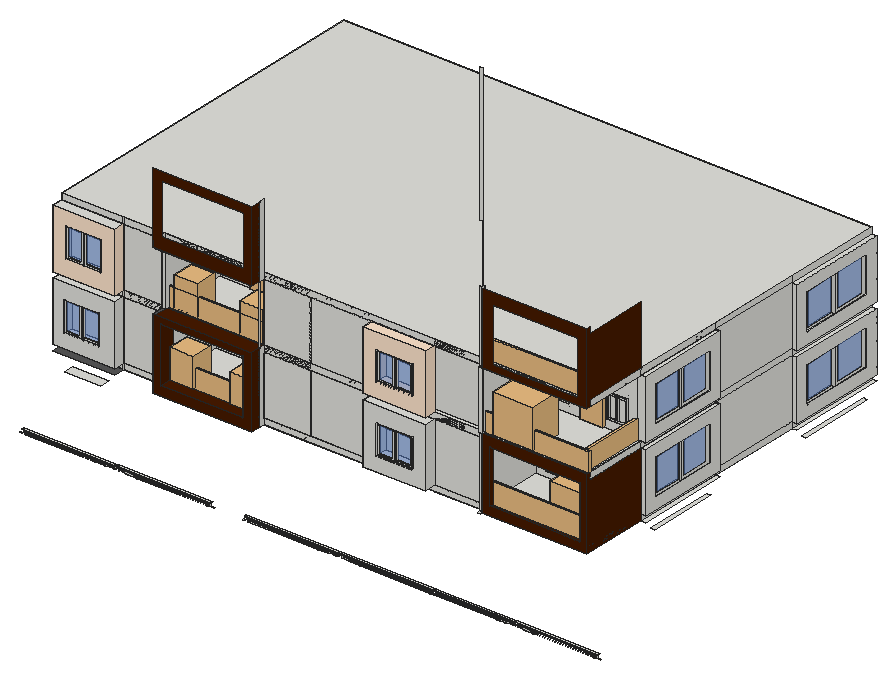
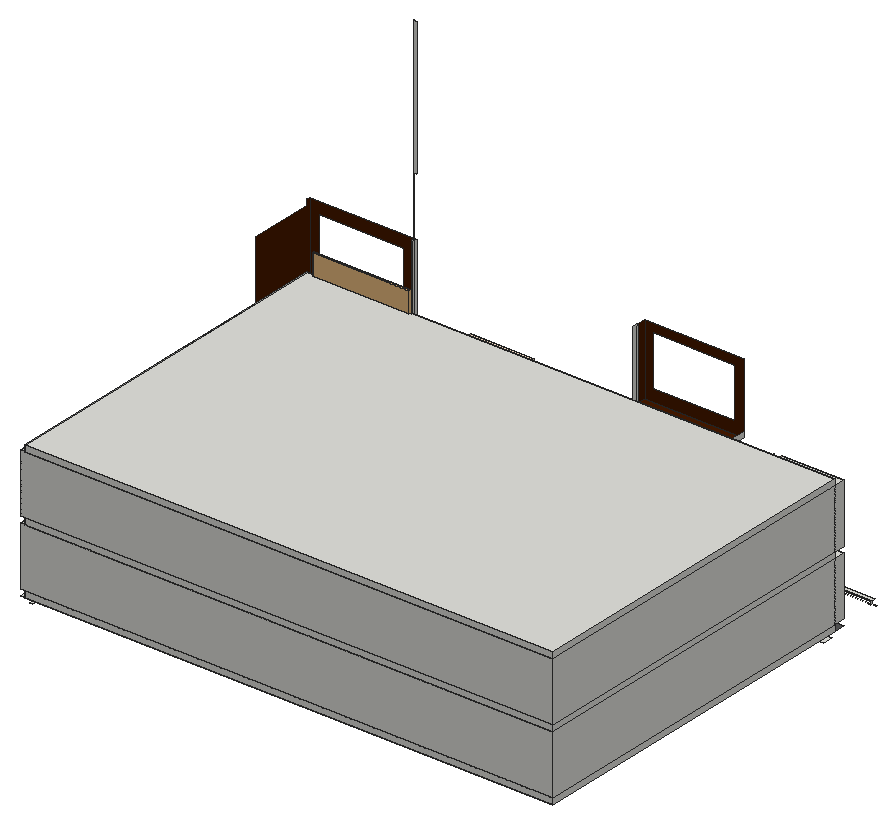
# SketchUp Ruby script. Lengths in inches.
U = 1.inch
M = Sketchup.active_model
def pt(a) = Geom::Point3d.new(a.map { |v| v * U })
def face(e, loops, mat)
  f = e.add_face(loops[0].map { |a| pt(a) })
  loops[1..].each { |l| e.add_face(l.map { |a| pt(a) }).erase! }
  f.material = f.back_material = mat if mat
  f
end
# faces: each face lists its corners as indices into pts; further lists are holes
def faces(e, pts, list, mat = nil) = list.each { |f| face(e, (f[0].is_a?(Array) ? f : [f]).map { |l| l.map { |i| pts[i] } }, mat) }
# xy, xz, yz: faces in a plane at the given z, y or x. An outline is a flat list of corners, or four numbers for a rectangle; further outlines are holes
def ring(l) = l.size == 4 ? [[l[0], l[1]], [l[2], l[1]], [l[2], l[3]], [l[0], l[3]]] : l.each_slice(2).to_a
def flat(e, list, mat, &to3) = list.each { |f| face(e, (f[0].is_a?(Array) ? f : [f]).map { |l| ring(l).map { |u, v| to3.(u, v) } }, mat) }
def xy(e, z, list, mat = nil) = flat(e, list, mat) { |x, y| [x, y, z] }
def xz(e, y, list, mat = nil) = flat(e, list, mat) { |x, z| [x, y, z] }
def yz(e, x, list, mat = nil) = flat(e, list, mat) { |y, z| [x, y, z] }
def lines(e, pts, list) = list.each { |a, b| e.add_line(pt(pts[a]), pt(pts[b])) }
# prism: a flat outline (further loops are holes) pulled along v
def prism(e, loops, v, mat = nil)
  f = face(e, loops, mat); d = Geom::Vector3d.new(v.map { |x| x * U })
  f.pushpull(f.normal.samedirection?(d) ? d.length : -d.length)
end
def box(e, o, s, mat = nil) = prism(e, [[o, [o[0] + s[0], o[1], o[2]], [o[0] + s[0], o[1] + s[1], o[2]], [o[0], o[1] + s[1], o[2]]]], [0, 0, s[2]], mat)
def at(x, y, z, deg = 0) = Geom::Transformation.translation(pt([x, y, z])) * Geom::Transformation.rotation(ORIGIN, Z_AXIS, deg.degrees)
def axes(o, x, y, z) = Geom::Transformation.new([*x, 0, *y, 0, *z, 0, *pt(o).to_a, 1])
def part(name) = M.definitions.add(name)
# library, detail: a bought-in or finely detailed component or shape, given as its bounding box
def library(name, o, s) = part(name).tap { |d| box(d.entities, o, s) }
def detail(e, o, s) = box(e.add_group.entities, o, s)
def put(e, d, t, mat = nil) = e.add_instance(d, t).tap { |i| i.material = mat if mat }
def group(e, t, mat = nil) = e.add_group.tap { |g| g.transformation = t; g.material = mat if mat }.entities
root = M.entities
M.materials.add("[Color C01]").color = [255, 229, 204]
M.materials.add("[Color C07]").color = [71, 27, 0]
M.materials.add("[Color M06]").color = [86, 86, 86]
M.materials.add("[Color_000]").color = [255, 255, 255]
M.materials.add("[Translucent Glass Blue]").color = [100, 149, 237]
M.materials["[Translucent Glass Blue]"].alpha = 0.5
c1 = library("porta 4",[0.2,-5.42,1.33],[46.55,4.72,83.21])
c2 = library("Glass balustrade section",[0,0,0],[60.75,3.875,44.35])
c3 = library("KentiaPalm",[-22.86,-14.31,0],[47.49,43.96,59.125])
c4 = library("Round Planter with Plant",[-35.48,-39.77,0],[80.62,63.55,77.875])
c5 = part("Window")
xy(c5.entities,31.72,[[-0.78,88.6,2.72,128.1]])
xy(c5.entities,34.95,[[-0.78,91.53,0.84,106.59],[0.84,91.53,1.05,97.58],[1.05,91.53,1.42,106.59],[1.42,91.53,2.72,106.59],[0.84,97.58,1.05,98.18],
  [0.84,98.18,1.05,106.59]])
xy(c5.entities,35.27,[[-0.78,110.09,0.97,125.14],[1.05,110.09,2.72,125.14]])
xy(c5.entities,58.35,[[2.72,108.74,3.8,109.74]])
xy(c5.entities,77.8125,[[-0.78,110.09,2.72,125.14],[0.97,110.09,1.05,125.14]])
xy(c5.entities,77.93,[[-0.78,91.53,0.84,106.59],[1.05,91.53,1.42,106.59],[1.42,91.53,2.72,106.59]])
xy(c5.entities,80.72,[[-0.78,88.6,2.72,128.1]])
xz(c5.entities,88.6,[[-0.78,31.72,2.72,80.72]])
xz(c5.entities,91.53,[[-0.78,34.95,0.84,77.93],[1.05,34.95,1.42,77.93],[1.42,34.95,2.72,77.93]])
xz(c5.entities,106.59,[[-0.78,34.95,0.84,77.93],[0.84,34.95,1.05,77.93],[0.84,34.95,2.72,77.93]])
xz(c5.entities,108.74,[[3.8,54.35,4.22,54.6,4.22,59.47,2.72,59.97,2.72,58.35,3.8,58.35]])
xz(c5.entities,109.74,[[3.8,54.35,3.8,58.35,2.72,58.35,2.72,59.97,4.22,59.47,4.22,54.6]])
xz(c5.entities,110.09,[[-0.78,35.27,0.97,77.8125],[1.05,35.27,2.72,77.8125]])
xz(c5.entities,125.14,[[-0.78,35.27,0.97,77.8125],[0.97,35.27,1.05,80.72],[1.05,35.27,2.72,77.8125]])
xz(c5.entities,128.1,[[-0.78,31.72,2.72,80.72]])
yz(c5.entities,-0.78,[[[88.6,31.72,128.1,80.72],[91.53,34.95,106.59,77.93],[110.09,35.27,125.14,77.8125]]])
yz(c5.entities,0.84,[[91.53,34.95,106.59,77.93]])
yz(c5.entities,0.97,[[110.09,35.27,125.14,77.8125]])
yz(c5.entities,1.05,[[91.53,34.95,106.59,77.93],[110.09,35.27,125.14,77.8125]])
yz(c5.entities,1.42,[[91.53,34.95,106.59,77.93]])
yz(c5.entities,2.72,[[[88.6,31.72,108.35,80.72],[91.53,34.95,106.59,77.93]],[[108.35,31.72,128.1,80.72],[110.09,35.27,125.14,77.8125],[108.74,58.35,109.74,59.97]]])
yz(c5.entities,3.8,[[108.74,54.35,109.74,58.35]])
yz(c5.entities,4.22,[[108.74,54.6,109.74,59.47]])
p = [[4.22,108.74,54.6],[3.8,108.74,54.35],[3.8,109.74,54.35],[4.22,109.74,54.6],[2.72,109.74,59.97],[2.72,108.74,59.97],
  [4.22,108.74,59.47],[4.22,109.74,59.47],[-0.78,86.4,89.94],[-0.78,86.44,89.94],[15.22,130.69,89.94],[15.22,130.65,89.94],
  [-0.78,86.44,28.19],[-0.78,86.4,28.19],[7.72,130.69,89.94],[7.72,130.65,89.94]]
faces(c5.entities,p,[[0,1,2,3],[4,5,6,7]])
lines(c5.entities,p,[[8,9],[10,11],[12,13],[14,15]])
c6 = part("Janela aluminio")
xy(c6.entities,0,[[0,0,47.24,1.57],[23.62,1.57,47.24,2.76],[0,2.76,25.98,3.9375],[0,3.9375,47.24,5.91]])
xy(c6.entities,43.31,[[0,0,47.24,1.57],[23.62,1.57,47.24,2.76],[0,2.76,0,5.91,47.24,5.91,47.24,3.9375,25.98,3.9375,25.98,2.76],[25.98,2.76,47.24,3.9375]])
xz(c6.entities,1.57,[[0,0,23.62,0,23.62,41.34,21.26,41.34,21.26,1.97,1.97,1.97,1.97,41.34,23.62,41.34,23.62,43.31,0,43.31],[[23.62,0,47.24,43.31],[25.7,1.97,45.28,41.34]]])
xz(c6.entities,2.76,[[[0,0,23.62,43.31],[2.36,2.36,21.26,40.94]],[23.62,0,25.98,43.31]])
xz(c6.entities,2.76,[[2.36,2.36,21.26,40.94]],"[Translucent Glass Blue]")
xz(c6.entities,3.9375,[[25.98,0,25.98,2.36,44.88,2.36,44.88,40.94,25.98,40.94,25.98,43.31,47.24,43.31,47.24,0]])
xz(c6.entities,3.9375,[[25.98,2.36,44.88,40.94]],"[Translucent Glass Blue]")
yz(c6.entities,0,[[0,0,1.57,43.31],[2.76,0,5.91,43.31]])
yz(c6.entities,23.62,[[1.57,0,2.76,43.31]])
yz(c6.entities,25.98,[[2.76,0,3.9375,43.31]])
yz(c6.entities,47.24,[[0,0,1.57,43.31],[1.57,0,2.76,43.31],[3.9375,0,5.91,43.31]])
xy(root,64.41,[[193.54,12.93,336.13,13.56],[336.13,12.93,354.73,13.56],[401.38,12.93,419.98,13.56],[419.98,12.93,562.58,13.56],[643.44,12.93,786.03,13.56],
  [786.03,12.93,804.64,13.56],[851.28,12.93,869.89,13.56],[869.89,12.93,1012.48,13.56],[1024.39,12.93,1148.45,13.56],[1148.45,12.93,1164.63,13.56],
  [1205.21,12.93,1221.4,13.56],[1221.4,12.93,1345.46,13.56],[193.54,13.81,336.13,14.31],[336.13,13.81,354.73,14.31],[401.38,13.81,419.98,14.31],
  [419.98,13.81,562.58,14.31],[643.44,13.81,786.03,14.31],[786.03,13.81,804.64,14.31],[851.28,13.81,869.89,14.31],[869.89,13.81,1012.48,14.31],
  [1024.39,13.81,1148.45,14.31],[1148.45,13.81,1164.63,14.31],[1205.21,13.81,1221.4,14.31],[1221.4,13.81,1345.46,14.31]])
xy(root,64.91,[[192.75,12.93,336.13,14.31],[336.13,12.93,355.52,14.31],[400.59,12.93,419.98,14.31],[419.98,12.93,563.36,14.31],[642.65,12.93,786.03,14.31],
  [786.03,12.93,805.43,14.31],[850.5,12.93,869.89,14.31],[869.89,12.93,1013.27,14.31],[1023.71,12.93,1148.45,14.31],[1148.45,12.93,1165.32,14.31],
  [1204.53,12.93,1221.4,14.31],[1221.4,12.93,1346.14,14.31]])
xy(root,64.96,[[182.38,13.24,186.86,14.43],[569.26,13.24,573.73,14.43],[632.29,13.24,636.76,14.43],[1014.6875,13.24,1018.58,14.43],[1019.16,13.24,1023.63,14.43],
  [1351.27,13.24,1355.16,14.43]])
xy(root,70.2,[[192.75,11.31,371.55,15.56],[384.5625,11.31,563.36,15.56],[642.65,11.31,821.45,15.56],[834.47,11.31,1013.27,15.56],[1023.71,11.31,1179.26,15.56],
  [1190.59,11.31,1346.14,15.56]])
xy(root,70.9,[[191.63,11.31,372.66,11.81],[383.45,11.31,564.48,11.81],[641.54,11.31,822.57,11.81],[833.35,11.31,1014.39,11.81],[1022.73,11.31,1180.23,11.81],
  [1189.61,11.31,1347.11,11.81],[191.63,14.12,372.66,15.56],[383.45,14.12,564.48,15.56],[641.54,14.12,822.57,15.56],[833.35,14.12,1014.39,15.56],
  [1022.73,14.12,1180.23,15.56],[1189.61,14.12,1347.11,15.56]])
xy(root,71.3,[[373.64,7.12,375.46,11.81],[380.65,7.12,382.48,11.81],[823.54,7.12,825.37,11.81],[830.56,7.12,832.38,11.81],[1181.08,7.12,1182.66,11.81],
  [1187.18,7.12,1188.77,11.81]],"[Color_000]")
xy(root,72.7,[[373.64,4.75,375.46,11.81],[380.65,4.75,382.48,11.81],[823.54,4.75,825.37,11.81],[830.56,4.75,832.38,11.81],[1181.08,4.75,1182.66,11.81],
  [1187.18,4.75,1188.77,11.81]],"[Color_000]")
xy(root,73.2,[[187.97,11.31,376.32,11.81],[379.79,11.31,568.14,11.81],[637.88,11.31,826.23,11.81],[829.7,11.31,1018.04,11.81],[1019.55,11.31,1183.41,11.81],
  [1186.43,11.31,1350.3,11.81],[187.97,14.12,376.32,15.56],[379.79,14.12,568.14,15.56],[637.88,14.12,826.23,15.56],[829.7,14.12,1018.04,15.56],
  [1019.55,14.12,1183.41,15.56],[1186.43,14.12,1350.3,15.56]])
xy(root,73.9,[[186.86,11.31,377.4375,15.56],[378.67,11.31,569.26,15.56],[636.76,11.31,827.35,15.56],[828.58,11.31,1019.16,15.56],[1018.58,11.31,1184.39,15.56],
  [1185.46,11.31,1351.27,15.56]])
xy(root,90.15,[[145.1,172.4375,217.17,193.125]])
xy(root,96.99,[[1188.1875,348.57,1196,490.48],[1188.1875,729.48,1196,885.06]])
xy(root,119.76,[[968.8125,186.3125,975.125,191.25]])
xy(root,120,[[974.8125,189.1875,1186.5,195.5625],[327.85,189.875,333.1,195.5625],[[119.8125,195.5625,333.1,195.5625,333.1,325.5625,528.67,325.5625,528.67,195.5625,974.8125,195.5625,974.8125,325.5625,1186.5,325.5625,1186.5,706.47,1196,706.47,1196,908.0625,119.8125,908.0625],[180.5,204.5625,180.5,894.25,1177.5,894.25,1177.5,334.5625,965.8125,334.5625,965.8125,204.5625,537.67,204.5625,537.67,334.5625,318.85,334.5625,318.85,204.5625]],[974.8125,195.5625,1186.5,325.5625],[1186.5,325.5625,1196,513.49]])
xy(root,120,[[333.1,165.375,528.5625,195.5625]],"[Color C07]")
xy(root,120,[[327.85,165.375,333.1,189.875],[119.8125,172.4375,244.96,195.5625]],"[Color M06]")
xy(root,132,[[119.8125,172.4375,244.96,195.5625],[[119.8125,195.5625,327.85,195.5625,327.85,325.5625,528.67,325.5625,528.67,195.5625,974.8125,195.5625,974.8125,325.5625,1186.5,325.5625,1186.5,706.47,1196,706.47,1196,908.0625,119.8125,908.0625],[180.5,204.5625,180.5,894.25,1177.5,894.25,1177.5,334.5625,965.8125,334.5625,965.8125,204.5625,537.67,204.5625,537.67,334.5625,318.85,334.5625,318.85,204.5625]],[327.85,195.5625,528.67,204.5625],[974.8125,195.5625,1172.34,204.5625],[180.5,204.5625,318.85,204.5625,318.85,334.5625,537.67,334.5625,537.67,204.5625,965.8125,204.5625,965.8125,334.5625,1177.5,334.5625,1177.5,894.25,180.5,894.25],
  [327.85,204.5625,528.67,325.5625],[974.8125,204.5625,1172.34,325.5625],[1172.34,204.5625,1177.5,325.5625],[1186.5,325.5625,1196,513.49]])
xy(root,137.5,[[990.52,189.1875,1172.34,195.5625]],"[Color C07]")
xy(root,139.0625,[[344.14,165.375,510.7,195.5625]],"[Color C07]")
xy(root,155.01,[[1188.1875,348.57,1196,490.48],[1188.1875,729.48,1196,885.06]])
xy(root,162.4,[[145.59,172.4375,214.55,188.9375]])
xy(root,221.6,[[145.59,172.4375,214.55,188.9375]])
xy(root,228.99,[[1188.1875,348.57,1196,490.48],[1188.1875,729.48,1196,885.06]])
xy(root,244.26,[[990.52,189.1875,1172.34,195.5625]],"[Color C07]")
xy(root,251.2,[[344.14,165.375,510.7,195.5625]],"[Color C07]")
xy(root,251.95,[[1172.34,195.5625,1186.5,325.5625]])
xy(root,252,[[119.8125,172.4375,244.96,195.5625],[[119.8125,195.5625,327.85,195.5625,327.85,325.5625,528.67,325.5625,528.67,195.5625,974.8125,195.5625,974.8125,325.5625,1186.5,325.5625,1186.5,706.47,1196,706.47,1196,908.0625,119.8125,908.0625],[180.5,204.5625,180.5,894.25,1177.5,894.25,1177.5,334.5625,965.8125,334.5625,965.8125,204.5625,537.67,204.5625,537.67,334.5625,318.85,334.5625,318.85,204.5625]],[1186.5,325.5625,1196,513.49]])
xy(root,264,[[119.8125,172.4375,244.96,195.5625],[974.8125,189.1875,1186.5,195.5625],[327.85,189.875,334.6,195.5625],[[119.8125,195.5625,334.6,195.5625,334.6,325.5625,528.67,325.5625,528.67,195.5625,974.8125,195.5625,974.8125,325.5625,1186.5,325.5625,1186.5,706.47,1196,706.47,1196,908.0625,119.8125,908.0625],[180.5,204.5625,180.5,894.25,1177.5,894.25,1177.5,334.5625,965.8125,334.5625,965.8125,204.5625,537.67,204.5625,537.67,334.5625,318.85,334.5625,318.85,204.5625]],[334.6,195.5625,528.67,204.5625],
  [974.8125,195.5625,1186.5,195.5625,1186.5,325.5625,1177.5,325.5625,1177.5,204.5625,974.8125,204.5625],[180.5,204.5625,318.85,204.5625,318.85,334.5625,537.67,334.5625,537.67,204.5625,965.8125,204.5625,965.8125,334.5625,1177.5,334.5625,1177.5,894.25,180.5,894.25],[334.6,204.5625,528.67,325.5625],[974.8125,204.5625,1177.5,325.5625],[1186.5,325.5625,1196,513.49]])
xy(root,264,[[334.6,165.375,528.5625,195.5625]],"[Color C07]")
xy(root,264,[[327.85,165.375,334.6,189.875]],"[Color M06]")
xy(root,264.21,[[968.8125,187.5625,975.125,191.25]])
xy(root,287.01,[[1188.1875,348.57,1196,490.48],[1188.1875,729.48,1196,885.06]])
xy(root,296.05,[[146.5625,172.4375,217.46,186.5]])
xy(root,356.5,[[146.5625,172.4375,217.46,186.5]])
xy(root,360.31,[[1188.1875,348.57,1196,348.76]])
xy(root,360.99,[[1188.1875,348.76,1196,490.48],[1188.1875,729.48,1196,885.06]])
xy(root,382.99,[[968.8125,187.5625,975.125,191.25]])
xy(root,383.3125,[[974.8125,188.8125,1186.5,195.5625],[1186.5,325.5625,1196,325.75]])
xy(root,384,[[327.85,165.375,334.6,189.875],[119.8125,172.4375,244.96,195.5625],[327.85,189.875,334.6,195.5625],[[119.8125,195.5625,334.6,195.5625,334.6,325.5625,528.67,325.5625,528.67,195.5625,974.8125,195.5625,974.8125,325.5625,1186.5,325.5625,1186.5,706.47,1196,706.47,1196,908.0625,119.8125,908.0625],[180.5,204.5625,180.5,894.25,1177.5,894.25,1177.5,334.5625,965.8125,334.5625,965.8125,204.5625,537.67,204.5625,537.67,334.5625,318.85,334.5625,318.85,204.5625]],[1186.5,325.75,1196,513.49]])
xy(root,384,[[334.6,165.375,528.5625,195.5625]],"[Color C07]")
xz(root,11.81,[[373.64,71.3,375.46,72.7],[380.65,71.3,382.48,72.7],[823.54,71.3,825.37,72.7],[830.56,71.3,832.38,72.7],[1181.08,71.3,1182.66,72.7],
  [1187.18,71.3,1188.77,72.7]],"[Color_000]")
xz(root,12.93,[[336.13,64.91,355.52,64.91,371.55,66.96,371.55,70.2,350.32,67.33,337.09,65.11],[400.59,64.91,384.5625,66.96,384.5625,70.2,405.79,67.33,419.02,65.11,419.98,64.91],[786.03,64.91,805.43,64.91,821.45,66.96,821.45,70.2,800.23,67.33,787,65.11],[850.5,64.91,834.47,66.96,834.47,70.2,855.7,67.33,868.93,65.11,869.89,64.91],[1148.45,64.91,1165.32,64.91,1179.26,66.96,1179.26,70.2,1160.8,67.33,1149.28,65.11],
  [1204.53,64.91,1190.59,66.96,1190.59,70.2,1209.05,67.33,1220.56,65.11,1221.4,64.91]])
xz(root,14.31,[[336.13,64.91,337.09,65.11,350.32,67.33,371.55,70.2,371.55,66.96,355.52,64.91],[400.59,64.91,419.98,64.91,419.02,65.11,405.79,67.33,384.5625,70.2,384.5625,66.96],[786.03,64.91,787,65.11,800.23,67.33,821.45,70.2,821.45,66.96,805.43,64.91],[850.5,64.91,869.89,64.91,868.93,65.11,855.7,67.33,834.47,70.2,834.47,66.96],[1148.45,64.91,1149.28,65.11,1160.8,67.33,1179.26,70.2,1179.26,66.96,1165.32,64.91],
  [1204.53,64.91,1221.4,64.91,1220.56,65.11,1209.05,67.33,1190.59,70.2,1190.59,66.96]])
xz(root,165.375,[[[327.85,120,528.5625,264],[344.14,139.0625,510.7,251.2]],[[327.85,384,528.5625,528],[345.85,408.8125,511.9375,510.75]]],"[Color C07]")
xz(root,172.4375,[[[119.8125,132,244.96,252],[145.59,162.4,214.55,221.6]]])
xz(root,172.4375,[[[119.8125,264,244.96,384],[146.5625,296.05,217.46,356.5]]],"[Color C01]")
xz(root,186.5,[[146.5625,296.05,217.46,356.5]])
xz(root,187.5625,[[968.8125,264.21,975.125,382.99]])
xz(root,188.8125,[[[974.8125,383.3125,1186.5,528],[997.1,396,1167.48,504.25]]],"[Color C07]")
xz(root,188.9375,[[145.59,162.4,214.55,221.6]])
xz(root,189.1875,[[[974.8125,120,1186.5,264],[990.52,137.5,1172.34,244.26]]],"[Color C07]")
xz(root,189.875,[[327.85,264,334.6,384]])
xz(root,191.25,[[968.8125,119.76,975.125,264.21],[968.8125,382.99,975.125,382.99,975.125,924,968.8125,924,968.8125,647.61,974.8125,647.61,974.8125,528,968.8125,528]])
xz(root,195.5625,[[244.96,120,325.71,132],[327.85,120,528.5625,132],[528.67,120,620.44,132],[622.95,120,747.02,132],[873.5,120,974.8125,132],
  [119.8125,132,244.96,252],[244.96,132,325.71,252],[325.71,132,327.85,252],[327.85,132,327.85,264,528.5625,264,528.5625,132,510.7,132,510.7,251.2,344.14,251.2,344.14,132],[344.14,132,510.7,139.0625],
  [528.67,132,620.44,252],[620.44,132,622.95,252],[622.95,132,747.02,252],[747.02,132,873.5,252],[873.5,132,974.8125,252],
  [974.8125,132,974.8125,264,1186.5,264,1186.5,251.95,1172.34,251.95,1172.34,244.26,990.52,244.26,990.52,132],[990.52,132,1172.34,137.5],[244.96,252,325.71,264],[528.67,252,620.44,264],[622.95,252,747.02,264],
  [873.5,252,974.8125,264],[119.8125,264,244.96,384],[244.96,264,325.71,384],[325.71,264,327.85,384],[528.67,264,620.44,384],
  [620.44,264,622.95,384],[622.95,264,747.02,384],[747.02,264,873.5,384],[974.8125,383.3125,1186.5,396],[244.96,384,325.71,396],
  [327.85,384,528.5625,396],[528.67,384,620.44,396],[622.95,384,747.02,396],[873.5,384,974.8125,396]])
xz(root,204.5625,[[180.5,132,318.85,252],[537.67,132,965.8125,252],[180.5,264,318.85,384],[537.67,264,965.8125,384]])
xz(root,325.5625,[[327.85,132,528.67,252],[974.8125,132,1172.34,132,1172.34,251.95,1177.5,251.95,1177.5,252,974.8125,252],[1172.34,132,1177.5,251.95],[1177.5,132,1186.5,251.95],[1186.5,132,1196,251.95],
  [1177.5,251.95,1186.5,252],[1186.5,251.95,1196,252],[334.6,264,528.67,384],[974.8125,264,1177.5,384],[1177.5,264,1186.5,264,1186.5,264.04,1196,264.04,1196,383.3125,1186.5,383.3125,1186.5,384,1177.5,384],
  [1186.5,264,1196,264.04]])
xz(root,325.75,[[1186.5,383.3125,1196,384]])
xz(root,334.5625,[[318.85,132,537.67,252],[965.8125,132,1177.5,252],[318.85,264,537.67,384],[965.8125,264,1177.5,384]])
xz(root,348.57,[[1188.1875,155.01,1196,228.99],[1188.1875,287.01,1196,360.31]])
xz(root,348.76,[[1188.1875,360.31,1196,360.99]])
xz(root,490.48,[[1188.1875,155.01,1196,228.99],[1188.1875,287.01,1196,360.99]])
xz(root,513.49,[[1186.5,132,1196,252],[1186.5,264,1196,384]])
xz(root,706.47,[[1186.5,132,1196,252],[1186.5,264,1196,384]])
xz(root,729.48,[[1188.1875,155.01,1196,228.99],[1188.1875,287.01,1196,360.99]])
xz(root,885.06,[[1188.1875,155.01,1196,228.99],[1188.1875,287.01,1196,360.99]])
xz(root,894.25,[[180.5,132,1177.5,252],[180.5,264,1177.5,384]])
xz(root,908.0625,[[119.8125,132,1196,252],[119.8125,264,1196,384]])
yz(root,119.8125,[[172.4375,132,195.5625,252],[195.5625,132,908.0625,252],[172.4375,264,195.5625,384],[195.5625,264,908.0625,384]])
yz(root,145.59,[[172.4375,162.4,188.9375,221.6]])
yz(root,146.5625,[[172.4375,296.05,186.5,356.5]])
yz(root,180.5,[[204.5625,132,894.25,252],[204.5625,264,894.25,384]])
yz(root,191.63,[[14.12,64.91,15.56,70.9]])
yz(root,214.55,[[172.4375,162.4,188.9375,221.6]])
yz(root,217.46,[[172.4375,296.05,186.5,356.5]])
yz(root,244.96,[[193.5625,120,195.5625,132],[172.4375,132,193.5625,252],[193.5625,132,195.5625,252],[193.5625,252,195.5625,264],[193.5625,264,195.5625,384],
  [193.5625,384,195.5625,396]])
yz(root,244.96,[[172.4375,264,193.5625,384]],"[Color C01]")
yz(root,318.85,[[204.5625,132,334.5625,252],[204.5625,264,334.5625,384]])
yz(root,327.85,[[165.375,120,195.5625,132],[165.375,132,195.5625,264],[195.5625,132,204.5625,252],[204.5625,132,325.5625,252],[189.875,264,195.5625,384],
  [165.375,384,195.5625,396]])
yz(root,334.6,[[189.875,264,325.5625,384]])
yz(root,344.14,[[165.375,139.0625,195.5625,251.2]],"[Color C07]")
yz(root,371.55,[[11.31,66.96,12.93,70.2],[14.31,66.96,15.56,70.2]])
yz(root,372.66,[[11.31,66.96,11.81,70.9],[14.12,66.96,15.56,70.9]])
yz(root,383.45,[[11.31,66.96,11.81,70.9],[14.12,66.96,15.56,70.9]])
yz(root,384.5625,[[11.31,66.96,12.93,70.2],[14.31,66.96,15.56,70.2]])
yz(root,510.7,[[165.375,139.0625,195.5625,251.2]])
yz(root,528.5625,[[182.3125,120,184.75,264],[184.75,120,195.5625,264],[182.3125,264,184.75,384],[182.3125,384,184.75,528],[184.75,384,195.5625,528]])
yz(root,528.5625,[[165.375,120,182.3125,264],[165.375,384,182.3125,528]],"[Color C07]")
yz(root,528.67,[[195.5625,132,204.5625,252],[204.5625,132,325.5625,252],[195.5625,264,204.5625,384],[204.5625,264,325.5625,384]])
yz(root,537.67,[[204.5625,132,334.5625,252],[204.5625,264,334.5625,384]])
yz(root,564.48,[[14.12,64.91,15.56,70.9]])
yz(root,641.54,[[14.12,64.91,15.56,70.9]])
yz(root,821.45,[[11.31,66.96,12.93,70.2],[14.31,66.96,15.56,70.2]])
yz(root,822.57,[[11.31,66.96,11.81,70.9],[14.12,66.96,15.56,70.9]])
yz(root,833.35,[[11.31,66.96,11.81,70.9],[14.12,66.96,15.56,70.9]])
yz(root,834.47,[[11.31,66.96,12.93,70.2],[14.31,66.96,15.56,70.2]])
yz(root,965.8125,[[204.5625,132,334.5625,252],[204.5625,264,334.5625,384]])
yz(root,974.8125,[[189.1875,120,193.6875,132],[193.6875,120,195.5625,132],[189.1875,132,193.6875,264],[193.6875,132,195.5625,264],[195.5625,132,204.5625,252],
  [204.5625,132,325.5625,252],[193.6875,264,325.5625,264,325.5625,384,195.5625,384,195.5625,383.3125,193.6875,383.3125],[188.8125,383.3125,193.6875,528],[193.6875,383.3125,195.5625,528]])
yz(root,990.52,[[189.1875,137.5,195.5625,244.26]],"[Color C07]")
yz(root,1014.39,[[14.12,64.91,15.56,70.9]])
yz(root,1022.73,[[14.12,64.91,15.56,70.9]])
yz(root,1172.34,[[195.5625,132,195.5625,137.5,189.1875,137.5,189.1875,244.26,195.5625,244.26,195.5625,251.95,325.5625,251.95,325.5625,132]])
yz(root,1177.5,[[334.5625,132,894.25,252],[334.5625,264,894.25,384]])
yz(root,1179.26,[[11.31,66.96,12.93,70.2],[14.31,66.96,15.56,70.2]])
yz(root,1180.23,[[11.31,66.96,11.81,70.9],[14.12,66.96,15.56,70.9]])
yz(root,1186.5,[[325.5625,120,513.49,132],[513.49,120,706.47,132],[513.49,132,706.47,252],[325.5625,252,513.49,264],[513.49,252,706.47,264],
  [513.49,264,706.47,384],[325.5625,383.3125,325.75,384],[325.75,384,513.49,396],[513.49,384,706.47,396]])
yz(root,1186.5,[[189.1875,120,325.5625,120,325.5625,251.95,195.5625,251.95,195.5625,264,189.1875,264],[195.5625,251.95,325.5625,264],[188.8125,383.3125,195.5625,383.3125,195.5625,396,325.5625,396,325.5625,516,195.5625,516,195.5625,528,188.8125,528],[195.5625,383.3125,325.5625,383.3125,325.5625,384,325.75,384,325.75,396,195.5625,396]],"[Color C07]")
yz(root,1188.1875,[[348.57,155.01,490.48,228.99],[729.48,155.01,885.06,228.99],[348.57,287.01,490.48,287.01,490.48,360.99,348.76,360.99,348.76,360.31,348.57,360.31],[729.48,287.01,885.06,360.99]])
yz(root,1189.61,[[11.31,66.96,11.81,70.9],[14.12,66.96,15.56,70.9]])
yz(root,1190.59,[[11.31,66.96,12.93,70.2],[14.31,66.96,15.56,70.2]])
yz(root,1196,[[[325.5625,132,513.49,252],[348.57,155.01,490.48,228.99]],[[706.47,132,908.0625,252],[729.48,155.01,885.06,228.99]],[[325.5625,264,513.49,264,513.49,384,325.75,384,325.75,383.3125,325.5625,383.3125],[348.57,287.01,348.57,360.31,348.76,360.31,348.76,360.99,490.48,360.99,490.48,287.01]],[[706.47,264,908.0625,384],[729.48,287.01,885.06,360.99]]])
yz(root,1347.11,[[14.12,64.91,15.56,70.9]])
p = [[337.09,14.31,65.11],[336.13,14.31,64.91],[336.13,12.93,64.91],[337.09,12.93,65.11],[355.52,14.31,64.91],[371.55,14.31,66.96],
  [371.55,12.93,66.96],[355.52,12.93,64.91],[400.59,14.31,64.91],[384.5625,14.31,66.96],[384.5625,12.93,66.96],[400.59,12.93,64.91],
  [419.02,14.31,65.11],[419.98,14.31,64.91],[419.98,12.93,64.91],[419.02,12.93,65.11],[787,14.31,65.11],[786.03,14.31,64.91],
  [786.03,12.93,64.91],[787,12.93,65.11],[805.43,14.31,64.91],[821.45,14.31,66.96],[821.45,12.93,66.96],[805.43,12.93,64.91],
  [850.5,14.31,64.91],[834.47,14.31,66.96],[834.47,12.93,66.96],[850.5,12.93,64.91],[868.93,14.31,65.11],[869.89,14.31,64.91],
  [869.89,12.93,64.91],[868.93,12.93,65.11],[1149.28,14.31,65.11],[1148.45,14.31,64.91],[1148.45,12.93,64.91],[1149.28,12.93,65.11],
  [1165.32,14.31,64.91],[1179.26,14.31,66.96],[1179.26,12.93,66.96],[1165.32,12.93,64.91],[1204.53,14.31,64.91],[1190.59,14.31,66.96],
  [1190.59,12.93,66.96],[1204.53,12.93,64.91],[1220.56,14.31,65.11],[1221.4,14.31,64.91],[1221.4,12.93,64.91],[1220.56,12.93,65.11],
  [350.32,14.31,67.33],[350.32,12.93,67.33],[405.79,14.31,67.33],[405.79,12.93,67.33],[800.23,14.31,67.33],[800.23,12.93,67.33],
  [855.7,14.31,67.33],[855.7,12.93,67.33],[1160.8,14.31,67.33],[1160.8,12.93,67.33],[1209.05,14.31,67.33],[1209.05,12.93,67.33],
  [371.55,14.31,70.2],[371.55,12.93,70.2],[384.5625,14.31,70.2],[384.5625,12.93,70.2],[821.45,14.31,70.2],[821.45,12.93,70.2],
  [834.47,14.31,70.2],[834.47,12.93,70.2],[1179.26,14.31,70.2],[1179.26,12.93,70.2],[1190.59,14.31,70.2],[1190.59,12.93,70.2],
  [1183.88,196.57,252],[1186.5,325.5625,252],[1186.5,325.5625,264],[1186.5,325.5625,264.04],[1183.88,196.57,264.04],[1186.5,195.5625,132],
  [1172.34,195.5625,132]]
faces(root,p,[[0,1,2,3],[4,5,6,7],[8,9,10,11],[12,13,14,15],[16,17,18,19],[20,21,22,23],[24,25,26,27],[28,29,30,31],
  [32,33,34,35],[36,37,38,39],[40,41,42,43],[44,45,46,47],[48,0,3,49],[50,12,15,51],[52,16,19,53],[54,28,31,55],
  [56,32,35,57],[58,44,47,59],[60,48,49,61],[62,50,51,63],[64,52,53,65],[66,54,55,67],[68,56,57,69],[70,58,59,71],
  [72,73,74,75,76]])
lines(root,p,[[77,78]])
g1 = group(root,at(171.4375,908.0625,120))
box(g1,[-51.625,-712.5,0],[1066.6875,712.5,12])
g2 = group(root,at(747.02,195.5625,131.3125))
xy(g2,0,[[0,-23.125,126.48,0]])
xy(g2,30.18,[[27.3,-23.125,100.24,0]])
xy(g2,88.07,[[27.3,-23.125,100.24,0]])
xy(g2,120,[[0,-23.125,126.48,0]])
xz(g2,-23.125,[[[0,0,126.48,120],[27.3,30.18,100.24,88.07]]])
xz(g2,0,[[[0,0,126.48,120],[27.3,30.18,100.24,88.07]],[27.3,30.18,100.24,88.07]])
yz(g2,0,[[-23.125,0,0,120]])
yz(g2,27.3,[[-23.125,30.18,0,88.07]])
yz(g2,100.24,[[-23.125,30.18,0,88.07]])
yz(g2,126.48,[[-23.125,0,0,120]])
put(root,c1,at(1067.5625,325.5625,130.36))
put(root,c1,at(400.125,325.5625,130.36))
put(root,c2,axes([331.61,190.625,133.125],[3.03753,0,0],[0,1,0],[0,0,1]),"[Color C07]")
put(root,c2,axes([977.8,195.5625,134.6875],[3.2022,0,0],[0,1,0],[0,0,1]))
put(root,c3,at(487.65,203,137.8))
put(root,c4,at(1137.72,241.32,139.15))
put(root,c3,at(368.49,200.09,141.05))
put(root,c5,at(1131.67,314.34,119.36,90))
put(root,c5,at(1249.11,314.34,119.36,90))
put(root,c5,at(475.11,314.34,119.36,90))
put(root,c5,at(592.54,314.34,119.36,90))
put(root,c6,axes([1188.68,490.48,155.01],[0,-2.99951,0],[1.24,0,0],[0,0,1.70845]))
put(root,c6,axes([1188.68,885.06,155.01],[0,-3.30143,0],[1.24,0,0],[0,0,1.70845]))
put(root,c6,axes([142.49,172.4375,161.14],[1.5254,0,0],[0,1,0],[0,0,1.39595]))
put(root,c6,axes([775.19,171.02,161.49],[1.5254,0,0],[0,1.24,0],[0,0,1.33678]))
g3 = group(root,at(171.4375,908.0625,252))
box(g3,[-51.625,-712.5,0],[1066.6875,712.5,12])
put(root,c2,axes([1172.45,334.48,257.7],[0,-2.16255,0],[1.77,0,0],[0,0,0.9879]))
put(root,c2,axes([969.17,194.8125,257.82],[3.57272,0,0],[0,1,0],[0,0,1]))
put(root,c2,axes([320.66,197.45,258.375],[3.42226,0,0],[0,1,0],[0,0,1]))
g4 = group(root,at(747.02,195.5625,264),"[Color C01]")
xy(g4,0,[[0,-23.125,126.48,0]])
xy(g4,31.24,[[28.18,-23.125,100.24,0]])
xy(g4,88.26,[[28.18,-23.125,100.24,0]])
xy(g4,120,[[0,-23.125,126.48,0]])
xz(g4,-23.125,[[[0,0,126.48,120],[28.18,31.24,100.24,88.26]]])
xz(g4,0,[[[0,0,126.48,120],[28.18,31.24,100.24,88.26]],[28.18,31.24,100.24,88.26]])
yz(g4,0,[[-23.125,0,0,120]])
yz(g4,28.18,[[-23.125,31.24,0,88.26]])
yz(g4,100.24,[[-23.125,31.24,0,88.26]])
yz(g4,126.48,[[-23.125,0,0,120]])
put(root,c4,at(1028.49,233.14,265.79))
put(root,c1,at(1067.5625,325.5625,264.62))
put(root,c1,at(400.125,325.5625,264.62))
put(root,c3,at(500.74,212.09,266.98))
put(root,c3,at(368.49,212.09,266.98))
put(root,c5,at(1249.11,323.03,250.93,90))
put(root,c5,at(1131.67,323.03,250.93,90))
put(root,c5,at(475.11,323.03,250.93,90))
put(root,c5,at(592.54,323.03,250.93,90))
put(root,c6,axes([1188.68,490.48,287.01],[0,-2.99951,0],[1.24,0,0],[0,0,1.70845]))
put(root,c6,axes([1188.68,885.06,287.01],[0,-3.30143,0],[1.24,0,0],[0,0,1.70845]))
put(root,c6,axes([775.19,171.02,294.37],[1.5254,0,0],[0,1.24,0],[0,0,1.33678]))
put(root,c6,axes([146.5625,172.4375,296.05],[1.5254,0,0],[0,1,0],[0,0,1.39595]))
g5 = group(root,at(171.4375,908.0625,384))
box(g5,[-51.625,-712.5,0],[1066.6875,712.5,12])
put(root,c2,axes([977.8,195.5625,393.0625],[3.2022,0,0],[0,1,0],[0,0,1]))
